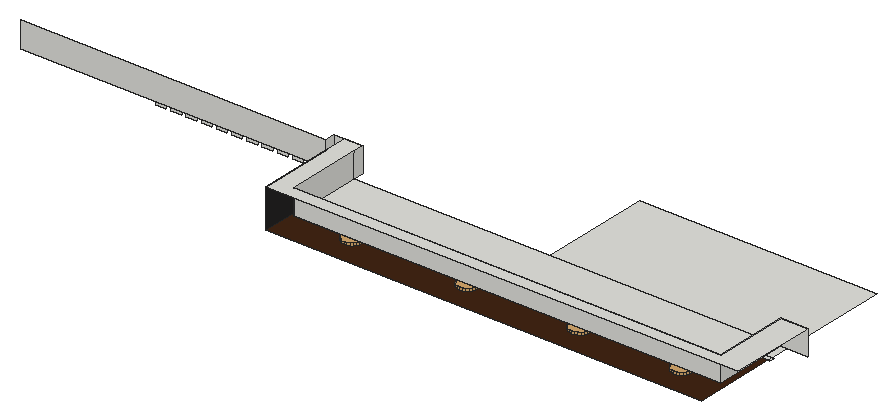
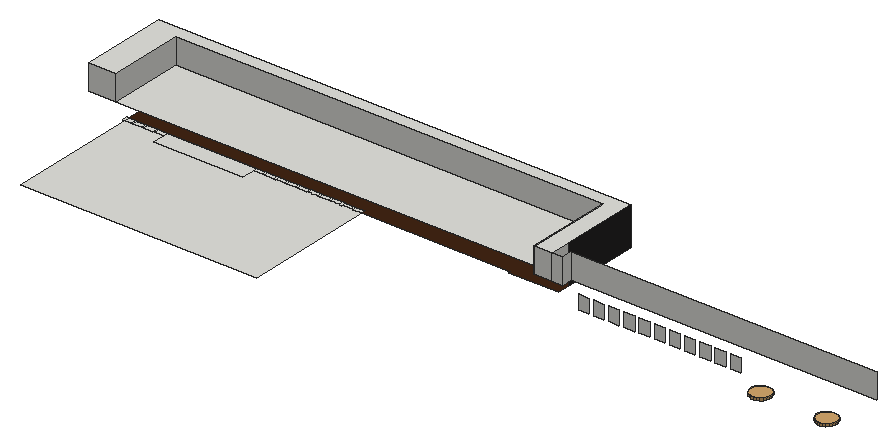
# SketchUp Ruby script. Lengths in inches.
U = 1.inch
M = Sketchup.active_model
def pt(a) = Geom::Point3d.new(a.map { |v| v * U })
def face(e, loops, mat)
  f = e.add_face(loops[0].map { |a| pt(a) })
  loops[1..].each { |l| e.add_face(l.map { |a| pt(a) }).erase! }
  f.material = f.back_material = mat if mat
  f
end
# faces: each face lists its corners as indices into pts; further lists are holes
def faces(e, pts, list, mat = nil) = list.each { |f| face(e, (f[0].is_a?(Array) ? f : [f]).map { |l| l.map { |i| pts[i] } }, mat) }
# xy, xz, yz: faces in a plane at the given z, y or x. An outline is a flat list of corners, or four numbers for a rectangle; further outlines are holes
def ring(l) = l.size == 4 ? [[l[0], l[1]], [l[2], l[1]], [l[2], l[3]], [l[0], l[3]]] : l.each_slice(2).to_a
def flat(e, list, mat, &to3) = list.each { |f| face(e, (f[0].is_a?(Array) ? f : [f]).map { |l| ring(l).map { |u, v| to3.(u, v) } }, mat) }
def xy(e, z, list, mat = nil) = flat(e, list, mat) { |x, y| [x, y, z] }
def xz(e, y, list, mat = nil) = flat(e, list, mat) { |x, z| [x, y, z] }
def yz(e, x, list, mat = nil) = flat(e, list, mat) { |y, z| [x, y, z] }
def lines(e, pts, list) = list.each { |a, b| e.add_line(pt(pts[a]), pt(pts[b])) }
# prism: a flat outline (further loops are holes) pulled along v
def prism(e, loops, v, mat = nil)
  f = face(e, loops, mat); d = Geom::Vector3d.new(v.map { |x| x * U })
  f.pushpull(f.normal.samedirection?(d) ? d.length : -d.length)
end
def box(e, o, s, mat = nil) = prism(e, [[o, [o[0] + s[0], o[1], o[2]], [o[0] + s[0], o[1] + s[1], o[2]], [o[0], o[1] + s[1], o[2]]]], [0, 0, s[2]], mat)
def at(x, y, z, deg = 0) = Geom::Transformation.translation(pt([x, y, z])) * Geom::Transformation.rotation(ORIGIN, Z_AXIS, deg.degrees)
def axes(o, x, y, z) = Geom::Transformation.new([*x, 0, *y, 0, *z, 0, *pt(o).to_a, 1])
def part(name) = M.definitions.add(name)
# library, detail: a bought-in or finely detailed component or shape, given as its bounding box
def library(name, o, s) = part(name).tap { |d| box(d.entities, o, s) }
def detail(e, o, s) = box(e.add_group.entities, o, s)
def put(e, d, t, mat = nil) = e.add_instance(d, t).tap { |i| i.material = mat if mat }
def group(e, t, mat = nil) = e.add_group.tap { |g| g.transformation = t; g.material = mat if mat }.entities
root = M.entities
M.materials.add("[Field Square Tile]").color = [211, 167, 108]
M.materials.add("[Granite Dark Gray]").color = [38, 37, 37]
M.materials.add("[Wood Veneer 01]").color = [66, 38, 20]
xy(root,380.5,[[2291.96,2343.96,2297.38,2346.71],[2297.38,2343.96,2298.58,2346.71],[2298.58,2343.96,2304.01,2346.71],[2304.01,2343.96,2305.21,2346.71],[2305.21,2343.96,2310.63,2346.71],
  [2310.63,2343.96,2311.83,2346.71],[2311.83,2343.96,2317.26,2346.71],[2317.26,2343.96,2318.46,2346.71],[2318.46,2343.96,2323.88,2346.71],[2323.88,2343.96,2325.08,2346.71],
  [2325.08,2343.96,2330.51,2346.71],[2330.51,2343.96,2331.71,2346.71],[2331.71,2343.96,2337.13,2346.71],[2337.13,2343.96,2338.33,2346.71],[2338.33,2343.96,2343.76,2346.71],
  [2343.76,2343.96,2344.96,2346.71],[2344.96,2343.96,2350.38,2346.71],[2350.38,2343.96,2351.58,2346.71],[2351.58,2343.96,2357.01,2346.71],[2357.01,2343.96,2410.56,2354.27],
  [2410.56,2343.96,2415.98,2346.71],[2415.98,2343.96,2417.18,2346.71],[2417.18,2343.96,2422.61,2346.71],[2422.61,2343.96,2423.81,2346.71],[2423.81,2343.96,2429.23,2346.71],
  [2429.23,2343.96,2430.06,2346.71],[2430.06,2343.96,2434.04,2346.71],[2434.04,2343.96,2435.48,2346.71],[2291.96,2346.71,2291.96,2425.46,2434.04,2425.46,2434.04,2346.71,2410.56,2346.71,2410.56,2354.27,2357.01,2354.27,2357.01,2346.71]])
xy(root,380.5,[[[2172.48,2294.125,2172.48,2347.9,2202.28,2347.9,2202.28,2346.71,2291.96,2346.71,2291.96,2343.96,2434.04,2343.96,2434.04,2294.125],[2407.83,2306.32,2409.39,2306.53,2410.83,2307.13,2412.08,2308.08,2413.03,2309.32,2413.63,2310.77,2413.83,2312.32,2413.63,2313.88,2413.03,2315.32,2412.08,2316.57,2410.83,2317.52,2409.39,2318.12,2407.83,2318.32,2406.28,2318.12,2404.83,2317.52,2403.59,2316.57,2402.64,2315.32,2402.04,2313.88,2401.83,2312.32,2402.04,2310.77,2402.64,2309.32,2403.59,2308.08,2404.83,2307.13,2406.28,2306.53],[2209.72,2306.32,2211.27,2306.53,2212.72,2307.13,2213.96,2308.08,2214.91,2309.32,2215.51,2310.77,2215.72,2312.32,2215.51,2313.88,2214.91,2315.32,2213.96,2316.57,2212.72,2317.52,2211.27,2318.12,2209.72,2318.32,2208.17,2318.12,2206.72,2317.52,2205.48,2316.57,2204.52,2315.32,2203.92,2313.88,2203.72,2312.32,2203.92,2310.77,2204.52,2309.32,2205.48,2308.08,2206.72,2307.13,2208.17,2306.53],[2279.18,2306.32,2280.73,2306.53,2282.18,2307.13,2283.42,2308.08,2284.38,2309.32,2284.98,2310.77,2285.18,2312.32,2284.98,2313.88,2284.38,2315.32,2283.42,2316.57,2282.18,2317.52,2280.73,2318.12,2279.18,2318.32,2277.63,2318.12,2276.18,2317.52,2274.9375,2316.57,2273.99,2315.32,2273.39,2313.88,2273.18,2312.32,2273.39,2310.77,2273.99,2309.32,2274.9375,2308.08,2276.18,2307.13,2277.63,2306.53],[2346.46,2306.32,2348.01,2306.53,2349.46,2307.13,2350.7,2308.08,2351.66,2309.32,2352.26,2310.77,2352.46,2312.32,2352.26,2313.88,2351.66,2315.32,2350.7,2316.57,2349.46,2317.52,2348.01,2318.12,2346.46,2318.32,2344.91,2318.12,2343.46,2317.52,2342.22,2316.57,2341.26,2315.32,2340.66,2313.88,2340.46,2312.32,2340.66,2310.77,2341.26,2309.32,2342.22,2308.08,2343.46,2307.13,2344.91,2306.53]]],"[Wood Veneer 01]")
xy(root,381.8125,[[2209.72,2306.32,2208.17,2306.53,2206.72,2307.13,2205.48,2308.08,2204.52,2309.32,2203.92,2310.77,2203.72,2312.32,2203.92,2313.88,2204.52,2315.32,2205.48,2316.57,2206.72,2317.52,2208.17,2318.12,2209.72,2318.32,2211.27,2318.12,2212.72,2317.52,2213.96,2316.57,2214.91,2315.32,2215.51,2313.88,2215.72,2312.32,2215.51,2310.77,2214.91,2309.32,2213.96,2308.08,2212.72,2307.13,2211.27,2306.53],[2279.18,2306.32,2277.63,2306.53,2276.18,2307.13,2274.9375,2308.08,2273.99,2309.32,2273.39,2310.77,2273.18,2312.32,2273.39,2313.88,2273.99,2315.32,2274.9375,2316.57,2276.18,2317.52,2277.63,2318.12,2279.18,2318.32,2280.73,2318.12,2282.18,2317.52,2283.42,2316.57,2284.38,2315.32,2284.98,2313.88,2285.18,2312.32,2284.98,2310.77,2284.38,2309.32,2283.42,2308.08,2282.18,2307.13,2280.73,2306.53],[2346.46,2306.32,2344.91,2306.53,2343.46,2307.13,2342.22,2308.08,2341.26,2309.32,2340.66,2310.77,2340.46,2312.32,2340.66,2313.88,2341.26,2315.32,2342.22,2316.57,2343.46,2317.52,2344.91,2318.12,2346.46,2318.32,2348.01,2318.12,2349.46,2317.52,2350.7,2316.57,2351.66,2315.32,2352.26,2313.88,2352.46,2312.32,2352.26,2310.77,2351.66,2309.32,2350.7,2308.08,2349.46,2307.13,2348.01,2306.53],[2407.83,2306.32,2406.28,2306.53,2404.83,2307.13,2403.59,2308.08,2402.64,2309.32,2402.04,2310.77,2401.83,2312.32,2402.04,2313.88,2402.64,2315.32,2403.59,2316.57,2404.83,2317.52,2406.28,2318.12,2407.83,2318.32,2409.39,2318.12,2410.83,2317.52,2412.08,2316.57,2413.03,2315.32,2413.63,2313.88,2413.83,2312.32,2413.63,2310.77,2413.03,2309.32,2412.08,2308.08,2410.83,2307.13,2409.39,2306.53]],"[Field Square Tile]")
xy(root,381.875,[[1998.33,2359.13,1996.77,2359.16,1995.26,2359.6,1993.92,2360.41,1992.84,2361.54,1992.08,2362.91,1991.71,2364.4375,1991.74,2366,1992.18,2367.51,1992.99,2368.85,1994.12,2369.93,1995.49,2370.69,1997.01,2371.06,1998.58,2371.03,2000.08,2370.59,2001.42,2369.78,2002.51,2368.65,2003.26,2367.28,2003.64,2365.75,2003.6,2364.1875,2003.17,2362.68,2002.36,2361.34,2001.23,2360.26,1999.85,2359.51],[2038.08,2359.13,2036.52,2359.16,2035.01,2359.6,2033.67,2360.41,2032.59,2361.54,2031.83,2362.91,2031.46,2364.4375,2031.49,2366,2031.93,2367.51,2032.74,2368.85,2033.87,2369.93,2035.24,2370.69,2036.76,2371.06,2038.33,2371.03,2039.83,2370.59,2041.17,2369.78,2042.26,2368.65,2043.01,2367.28,2043.39,2365.75,2043.35,2364.1875,2042.92,2362.68,2042.11,2361.34,2040.98,2360.26,2039.6,2359.51]],"[Field Square Tile]")
xy(root,388.625,[[2183.1875,2301.68,2439.68,2346.71]])
xy(root,403.8125,[[2172.48,2294.125,2455.66,2294.125,2455.66,2346.71,2439.68,2346.71,2439.68,2301.68,2183.1875,2301.68,2183.1875,2353.05,2172.48,2353.05]])
xz(root,2301.68,[[2183.1875,388.625,2439.68,403.8125]])
xz(root,2346.49,[[1982.81,388.625,2166.13,403.8125]])
xz(root,2346.71,[[2439.68,388.625,2455.66,403.8125]])
xz(root,2353.05,[[2166.13,388.625,2172.48,403.8125],[2172.48,388.625,2183.1875,403.8125]])
xz(root,2355.06,[[2057.43,380.5,2063.68,388.625],[2066.56,380.5,2072.81,388.625],[2075.68,380.5,2081.93,388.625],[2084.81,380.5,2091.06,388.625],[2093.93,380.5,2100.18,388.625],
  [2103.06,380.5,2109.31,388.625],[2112.18,380.5,2118.43,388.625],[2121.31,380.5,2127.56,388.625],[2130.43,380.5,2136.68,388.625],[2139.56,380.5,2145.81,388.625],
  [2148.68,380.5,2154.93,388.625]])
yz(root,2166.13,[[2346.49,388.625,2353.05,403.8125]])
yz(root,2172.48,[[2294.125,380.5,2340.15,403.8125]],"[Granite Dark Gray]")
yz(root,2183.1875,[[2301.68,388.625,2346.71,403.8125],[2346.71,388.625,2353.05,403.8125]])
yz(root,2439.68,[[2301.68,388.625,2346.71,403.8125]])
p = [[2209.72,2306.32,380.5],[2208.17,2306.53,380.5],[2208.17,2306.53,381.8125],[2209.72,2306.32,381.8125],[2211.27,2306.53,380.5],[2211.27,2306.53,381.8125],
  [2279.18,2306.32,380.5],[2277.63,2306.53,380.5],[2277.63,2306.53,381.8125],[2279.18,2306.32,381.8125],[2280.73,2306.53,380.5],[2280.73,2306.53,381.8125],
  [2346.46,2306.32,380.5],[2344.91,2306.53,380.5],[2344.91,2306.53,381.8125],[2346.46,2306.32,381.8125],[2348.01,2306.53,380.5],[2348.01,2306.53,381.8125],
  [2407.83,2306.32,380.5],[2406.28,2306.53,380.5],[2406.28,2306.53,381.8125],[2407.83,2306.32,381.8125],[2409.39,2306.53,380.5],[2409.39,2306.53,381.8125],
  [2206.72,2307.13,380.5],[2206.72,2307.13,381.8125],[2212.72,2307.13,380.5],[2212.72,2307.13,381.8125],[2276.18,2307.13,380.5],[2276.18,2307.13,381.8125],
  [2282.18,2307.13,380.5],[2282.18,2307.13,381.8125],[2343.46,2307.13,380.5],[2343.46,2307.13,381.8125],[2349.46,2307.13,380.5],[2349.46,2307.13,381.8125],
  [2404.83,2307.13,380.5],[2404.83,2307.13,381.8125],[2410.83,2307.13,380.5],[2410.83,2307.13,381.8125],[2205.48,2308.08,380.5],[2205.48,2308.08,381.8125],
  [2213.96,2308.08,380.5],[2213.96,2308.08,381.8125],[2274.9375,2308.08,380.5],[2274.9375,2308.08,381.8125],[2283.42,2308.08,380.5],[2283.42,2308.08,381.8125],
  [2342.22,2308.08,380.5],[2342.22,2308.08,381.8125],[2350.7,2308.08,380.5],[2350.7,2308.08,381.8125],[2403.59,2308.08,380.5],[2403.59,2308.08,381.8125],
  [2412.08,2308.08,380.5],[2412.08,2308.08,381.8125],[2204.52,2309.32,380.5],[2204.52,2309.32,381.8125],[2214.91,2309.32,380.5],[2214.91,2309.32,381.8125],
  [2273.99,2309.32,380.5],[2273.99,2309.32,381.8125],[2284.38,2309.32,380.5],[2284.38,2309.32,381.8125],[2341.26,2309.32,380.5],[2341.26,2309.32,381.8125],
  [2351.66,2309.32,380.5],[2351.66,2309.32,381.8125],[2402.64,2309.32,380.5],[2402.64,2309.32,381.8125],[2413.03,2309.32,380.5],[2413.03,2309.32,381.8125],
  [2203.92,2310.77,380.5],[2203.92,2310.77,381.8125],[2215.51,2310.77,380.5],[2215.51,2310.77,381.8125],[2273.39,2310.77,380.5],[2273.39,2310.77,381.8125],
  [2284.98,2310.77,380.5],[2284.98,2310.77,381.8125],[2340.66,2310.77,380.5],[2340.66,2310.77,381.8125],[2352.26,2310.77,380.5],[2352.26,2310.77,381.8125],
  [2402.04,2310.77,380.5],[2402.04,2310.77,381.8125],[2413.63,2310.77,380.5],[2413.63,2310.77,381.8125],[2203.72,2312.32,380.5],[2203.72,2312.32,381.8125],
  [2215.72,2312.32,380.5],[2215.72,2312.32,381.8125],[2273.18,2312.32,380.5],[2273.18,2312.32,381.8125],[2285.18,2312.32,380.5],[2285.18,2312.32,381.8125],
  [2340.46,2312.32,380.5],[2340.46,2312.32,381.8125],[2352.46,2312.32,380.5],[2352.46,2312.32,381.8125],[2401.83,2312.32,380.5],[2401.83,2312.32,381.8125],
  [2413.83,2312.32,380.5],[2413.83,2312.32,381.8125],[2203.92,2313.88,380.5],[2203.92,2313.88,381.8125],[2215.51,2313.88,380.5],[2215.51,2313.88,381.8125],
  [2273.39,2313.88,380.5],[2273.39,2313.88,381.8125],[2284.98,2313.88,380.5],[2284.98,2313.88,381.8125],[2340.66,2313.88,380.5],[2340.66,2313.88,381.8125],
  [2352.26,2313.88,380.5],[2352.26,2313.88,381.8125],[2402.04,2313.88,380.5],[2402.04,2313.88,381.8125],[2413.63,2313.88,380.5],[2413.63,2313.88,381.8125],
  [2204.52,2315.32,380.5],[2204.52,2315.32,381.8125],[2214.91,2315.32,380.5],[2214.91,2315.32,381.8125],[2273.99,2315.32,380.5],[2273.99,2315.32,381.8125],
  [2284.38,2315.32,380.5],[2284.38,2315.32,381.8125],[2341.26,2315.32,380.5],[2341.26,2315.32,381.8125],[2351.66,2315.32,380.5],[2351.66,2315.32,381.8125],
  [2402.64,2315.32,380.5],[2402.64,2315.32,381.8125],[2413.03,2315.32,380.5],[2413.03,2315.32,381.8125],[2205.48,2316.57,380.5],[2205.48,2316.57,381.8125],
  [2213.96,2316.57,380.5],[2213.96,2316.57,381.8125],[2274.9375,2316.57,380.5],[2274.9375,2316.57,381.8125],[2283.42,2316.57,380.5],[2283.42,2316.57,381.8125],
  [2342.22,2316.57,380.5],[2342.22,2316.57,381.8125],[2350.7,2316.57,380.5],[2350.7,2316.57,381.8125],[2403.59,2316.57,380.5],[2403.59,2316.57,381.8125],
  [2412.08,2316.57,380.5],[2412.08,2316.57,381.8125],[2206.72,2317.52,380.5],[2206.72,2317.52,381.8125],[2212.72,2317.52,380.5],[2212.72,2317.52,381.8125],
  [2276.18,2317.52,380.5],[2276.18,2317.52,381.8125],[2282.18,2317.52,380.5],[2282.18,2317.52,381.8125],[2343.46,2317.52,380.5],[2343.46,2317.52,381.8125],
  [2349.46,2317.52,380.5],[2349.46,2317.52,381.8125],[2404.83,2317.52,380.5],[2404.83,2317.52,381.8125],[2410.83,2317.52,380.5],[2410.83,2317.52,381.8125],
  [2208.17,2318.12,380.5],[2208.17,2318.12,381.8125],[2211.27,2318.12,380.5],[2211.27,2318.12,381.8125],[2277.63,2318.12,380.5],[2277.63,2318.12,381.8125],
  [2280.73,2318.12,380.5],[2280.73,2318.12,381.8125],[2344.91,2318.12,380.5],[2344.91,2318.12,381.8125],[2348.01,2318.12,380.5],[2348.01,2318.12,381.8125],
  [2406.28,2318.12,380.5],[2406.28,2318.12,381.8125],[2409.39,2318.12,380.5],[2409.39,2318.12,381.8125],[2209.72,2318.32,380.5],[2209.72,2318.32,381.8125],
  [2279.18,2318.32,380.5],[2279.18,2318.32,381.8125],[2346.46,2318.32,380.5],[2346.46,2318.32,381.8125],[2407.83,2318.32,380.5],[2407.83,2318.32,381.8125],
  [1998.33,2359.13,380.5],[1996.77,2359.16,380.5],[1996.77,2359.16,381.875],[1998.33,2359.13,381.875],[1999.85,2359.51,380.5],[1999.85,2359.51,381.875],
  [2038.08,2359.13,380.5],[2036.52,2359.16,380.5],[2036.52,2359.16,381.875],[2038.08,2359.13,381.875],[2039.6,2359.51,380.5],[2039.6,2359.51,381.875],
  [1995.26,2359.6,380.5],[1995.26,2359.6,381.875],[2035.01,2359.6,380.5],[2035.01,2359.6,381.875],[2001.23,2360.26,380.5],[2001.23,2360.26,381.875],
  [2040.98,2360.26,380.5],[2040.98,2360.26,381.875],[1993.92,2360.41,380.5],[1993.92,2360.41,381.875],[2033.67,2360.41,380.5],[2033.67,2360.41,381.875],
  [2002.36,2361.34,380.5],[2002.36,2361.34,381.875],[2042.11,2361.34,380.5],[2042.11,2361.34,381.875],[1992.84,2361.54,380.5],[1992.84,2361.54,381.875],
  [2032.59,2361.54,380.5],[2032.59,2361.54,381.875],[2003.17,2362.68,380.5],[2003.17,2362.68,381.875],[2042.92,2362.68,380.5],[2042.92,2362.68,381.875],
  [1992.08,2362.91,380.5],[1992.08,2362.91,381.875],[2031.83,2362.91,380.5],[2031.83,2362.91,381.875],[2003.6,2364.1875,380.5],[2003.6,2364.1875,381.875],
  [2043.35,2364.1875,380.5],[2043.35,2364.1875,381.875],[1991.71,2364.4375,380.5],[1991.71,2364.4375,381.875],[2031.46,2364.4375,380.5],[2031.46,2364.4375,381.875],
  [2003.64,2365.75,380.5],[2003.64,2365.75,381.875],[2043.39,2365.75,380.5],[2043.39,2365.75,381.875],[1991.74,2366,380.5],[1991.74,2366,381.875],
  [2031.49,2366,380.5],[2031.49,2366,381.875],[2003.26,2367.28,380.5],[2003.26,2367.28,381.875],[2043.01,2367.28,380.5],[2043.01,2367.28,381.875],
  [1992.18,2367.51,380.5],[1992.18,2367.51,381.875],[2031.93,2367.51,380.5],[2031.93,2367.51,381.875],[2002.51,2368.65,380.5],[2002.51,2368.65,381.875],
  [2042.26,2368.65,380.5],[2042.26,2368.65,381.875],[1992.99,2368.85,380.5],[1992.99,2368.85,381.875],[2032.74,2368.85,380.5],[2032.74,2368.85,381.875],
  [2001.42,2369.78,380.5],[2001.42,2369.78,381.875],[2041.17,2369.78,380.5],[2041.17,2369.78,381.875],[1994.12,2369.93,380.5],[1994.12,2369.93,381.875],
  [2033.87,2369.93,380.5],[2033.87,2369.93,381.875],[2000.08,2370.59,380.5],[2000.08,2370.59,381.875],[2039.83,2370.59,380.5],[2039.83,2370.59,381.875],
  [1995.49,2370.69,380.5],[1995.49,2370.69,381.875],[2035.24,2370.69,380.5],[2035.24,2370.69,381.875],[1998.58,2371.03,380.5],[1998.58,2371.03,381.875],
  [2038.33,2371.03,380.5],[2038.33,2371.03,381.875],[1997.01,2371.06,380.5],[1997.01,2371.06,381.875],[2036.76,2371.06,380.5],[2036.76,2371.06,381.875],
  [2172.5,2303.93,380.5],[2172.48,2294.125,380.5]]
faces(root,p,[[0,1,2,3],[4,0,3,5],[6,7,8,9],[10,6,9,11],[12,13,14,15],[16,12,15,17],[18,19,20,21],[22,18,21,23],
  [1,24,25,2],[26,4,5,27],[7,28,29,8],[30,10,11,31],[13,32,33,14],[34,16,17,35],[19,36,37,20],[38,22,23,39],
  [24,40,41,25],[42,26,27,43],[28,44,45,29],[46,30,31,47],[32,48,49,33],[50,34,35,51],[36,52,53,37],[54,38,39,55],
  [40,56,57,41],[58,42,43,59],[44,60,61,45],[62,46,47,63],[48,64,65,49],[66,50,51,67],[52,68,69,53],[70,54,55,71],
  [56,72,73,57],[74,58,59,75],[60,76,77,61],[78,62,63,79],[64,80,81,65],[82,66,67,83],[68,84,85,69],[86,70,71,87],
  [72,88,89,73],[90,74,75,91],[76,92,93,77],[94,78,79,95],[80,96,97,81],[98,82,83,99],[84,100,101,85],[102,86,87,103],
  [88,104,105,89],[106,90,91,107],[92,108,109,93],[110,94,95,111],[96,112,113,97],[114,98,99,115],[100,116,117,101],[118,102,103,119],
  [104,120,121,105],[122,106,107,123],[108,124,125,109],[126,110,111,127],[112,128,129,113],[130,114,115,131],[116,132,133,117],[134,118,119,135],
  [120,136,137,121],[138,122,123,139],[124,140,141,125],[142,126,127,143],[128,144,145,129],[146,130,131,147],[132,148,149,133],[150,134,135,151],
  [136,152,153,137],[154,138,139,155],[140,156,157,141],[158,142,143,159],[144,160,161,145],[162,146,147,163],[148,164,165,149],[166,150,151,167],
  [152,168,169,153],[170,154,155,171],[156,172,173,157],[174,158,159,175],[160,176,177,161],[178,162,163,179],[164,180,181,165],[182,166,167,183],
  [168,184,185,169],[184,170,171,185],[172,186,187,173],[186,174,175,187],[176,188,189,177],[188,178,179,189],[180,190,191,181],[190,182,183,191],
  [192,193,194,195],[196,192,195,197],[198,199,200,201],[202,198,201,203],[193,204,205,194],[199,206,207,200],[208,196,197,209],[210,202,203,211],
  [204,212,213,205],[206,214,215,207],[216,208,209,217],[218,210,211,219],[212,220,221,213],[214,222,223,215],[224,216,217,225],[226,218,219,227],
  [220,228,229,221],[222,230,231,223],[232,224,225,233],[234,226,227,235],[228,236,237,229],[230,238,239,231],[240,232,233,241],[242,234,235,243],
  [236,244,245,237],[238,246,247,239],[248,240,241,249],[250,242,243,251],[244,252,253,245],[246,254,255,247],[256,248,249,257],[258,250,251,259],
  [252,260,261,253],[254,262,263,255],[264,256,257,265],[266,258,259,267],[260,268,269,261],[262,270,271,263],[272,264,265,273],[274,266,267,275],
  [268,276,277,269],[270,278,279,271],[280,272,273,281],[282,274,275,283],[276,284,285,277],[278,286,287,279],[284,280,281,285],[286,282,283,287]],"[Field Square Tile]")
lines(root,p,[[288,289]])
